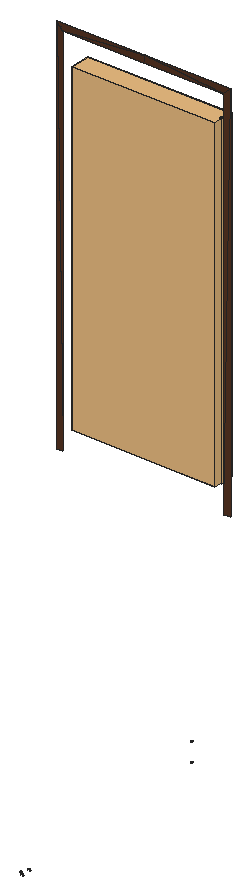
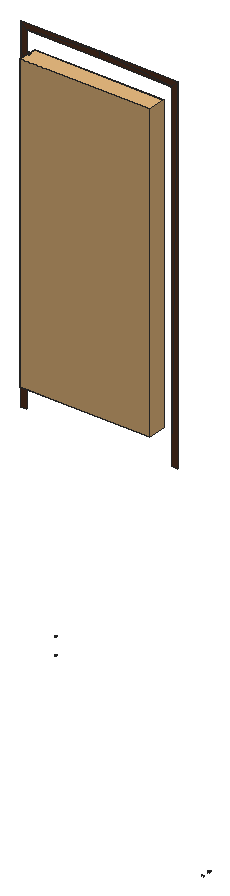
# SketchUp Ruby script. Lengths in inches.
U = 1.inch
M = Sketchup.active_model
def pt(a) = Geom::Point3d.new(a.map { |v| v * U })
def face(e, loops, mat)
  f = e.add_face(loops[0].map { |a| pt(a) })
  loops[1..].each { |l| e.add_face(l.map { |a| pt(a) }).erase! }
  f.material = f.back_material = mat if mat
  f
end
# faces: each face lists its corners as indices into pts; further lists are holes
def faces(e, pts, list, mat = nil) = list.each { |f| face(e, (f[0].is_a?(Array) ? f : [f]).map { |l| l.map { |i| pts[i] } }, mat) }
# xy, xz, yz: faces in a plane at the given z, y or x. An outline is a flat list of corners, or four numbers for a rectangle; further outlines are holes
def ring(l) = l.size == 4 ? [[l[0], l[1]], [l[2], l[1]], [l[2], l[3]], [l[0], l[3]]] : l.each_slice(2).to_a
def flat(e, list, mat, &to3) = list.each { |f| face(e, (f[0].is_a?(Array) ? f : [f]).map { |l| ring(l).map { |u, v| to3.(u, v) } }, mat) }
def xy(e, z, list, mat = nil) = flat(e, list, mat) { |x, y| [x, y, z] }
def xz(e, y, list, mat = nil) = flat(e, list, mat) { |x, z| [x, y, z] }
def yz(e, x, list, mat = nil) = flat(e, list, mat) { |y, z| [x, y, z] }
def lines(e, pts, list) = list.each { |a, b| e.add_line(pt(pts[a]), pt(pts[b])) }
# prism: a flat outline (further loops are holes) pulled along v
def prism(e, loops, v, mat = nil)
  f = face(e, loops, mat); d = Geom::Vector3d.new(v.map { |x| x * U })
  f.pushpull(f.normal.samedirection?(d) ? d.length : -d.length)
end
def box(e, o, s, mat = nil) = prism(e, [[o, [o[0] + s[0], o[1], o[2]], [o[0] + s[0], o[1] + s[1], o[2]], [o[0], o[1] + s[1], o[2]]]], [0, 0, s[2]], mat)
def at(x, y, z, deg = 0) = Geom::Transformation.translation(pt([x, y, z])) * Geom::Transformation.rotation(ORIGIN, Z_AXIS, deg.degrees)
def axes(o, x, y, z) = Geom::Transformation.new([*x, 0, *y, 0, *z, 0, *pt(o).to_a, 1])
def part(name) = M.definitions.add(name)
# library, detail: a bought-in or finely detailed component or shape, given as its bounding box
def library(name, o, s) = part(name).tap { |d| box(d.entities, o, s) }
def detail(e, o, s) = box(e.add_group.entities, o, s)
def put(e, d, t, mat = nil) = e.add_instance(d, t).tap { |i| i.material = mat if mat }
def group(e, t, mat = nil) = e.add_group.tap { |g| g.transformation = t; g.material = mat if mat }.entities
root = M.entities
M.materials.add("Material \#0").color = [86, 53, 35]
M.materials.add("Material \#1").color = [140, 140, 140]
c1 = library("3DGeom~9_Defintion",[456.52,-471.89,-18.89],[5.57,1000,5.49])
c2 = library("3DGeom~7_Defintion",[455.56,-471.94,-18.85],[5.55,1000,5.48])
c3 = part("3DGeom~8_Defintion")
xz(c3.entities,-471.94,[[458.125,-17.29,459.53,-16.11,457.73,-17.15],[458.125,-17.29,458.54,-17.29,459.53,-16.11],[458.54,-17.29,458.93,-17.15,459.53,-16.11],[457.73,-17.15,459.53,-16.11,457.42,-16.88],[458.93,-17.15,459.25,-16.88,459.53,-16.11],
  [457.42,-16.88,459.53,-16.11,457.21,-16.52],[459.25,-16.88,459.46,-16.52,459.53,-16.11],[457.21,-16.52,459.53,-16.11,457.14,-16.11],[457.14,-16.11,459.53,-16.11,457.21,-15.7],[459.53,-16.11,457.42,-15.34,457.21,-15.7],
  [459.53,-16.11,457.73,-15.07,457.42,-15.34],[459.53,-16.11,458.125,-14.93,457.73,-15.07],[459.53,-16.11,458.54,-14.93,458.125,-14.93],[459.53,-16.11,458.93,-15.07,458.54,-14.93],[459.53,-16.11,459.25,-15.34,458.93,-15.07],
  [459.53,-16.11,459.46,-15.7,459.25,-15.34]],"Material \#1")
xz(c3.entities,-416.39,[[458.125,-17.29,457.73,-17.15,459.53,-16.11],[458.125,-17.29,459.53,-16.11,458.54,-17.29],[458.54,-17.29,459.53,-16.11,458.93,-17.15],[457.73,-17.15,457.42,-16.88,459.53,-16.11],[458.93,-17.15,459.53,-16.11,459.25,-16.88],
  [457.42,-16.88,457.21,-16.52,459.53,-16.11],[459.25,-16.88,459.53,-16.11,459.46,-16.52],[457.21,-16.52,457.14,-16.11,459.53,-16.11],[457.14,-16.11,457.21,-15.7,459.53,-16.11],[459.53,-16.11,457.21,-15.7,457.42,-15.34],
  [459.53,-16.11,457.42,-15.34,457.73,-15.07],[459.53,-16.11,457.73,-15.07,458.125,-14.93],[459.53,-16.11,458.125,-14.93,458.54,-14.93],[459.53,-16.11,458.54,-14.93,458.93,-15.07],[459.53,-16.11,458.93,-15.07,459.25,-15.34],
  [459.53,-16.11,459.25,-15.34,459.46,-15.7]],"Material \#1")
xz(c3.entities,-27.5,[[458.125,-17.29,459.53,-16.11,457.73,-17.15],[458.125,-17.29,458.54,-17.29,459.53,-16.11],[458.54,-17.29,458.93,-17.15,459.53,-16.11],[457.73,-17.15,459.53,-16.11,457.42,-16.88],[458.93,-17.15,459.25,-16.88,459.53,-16.11],
  [457.42,-16.88,459.53,-16.11,457.21,-16.52],[459.25,-16.88,459.46,-16.52,459.53,-16.11],[457.21,-16.52,459.53,-16.11,457.14,-16.11],[457.14,-16.11,459.53,-16.11,457.21,-15.7],[459.53,-16.11,457.42,-15.34,457.21,-15.7],
  [459.53,-16.11,457.73,-15.07,457.42,-15.34],[459.53,-16.11,458.125,-14.93,457.73,-15.07],[459.53,-16.11,458.54,-14.93,458.125,-14.93],[459.53,-16.11,458.93,-15.07,458.54,-14.93],[459.53,-16.11,459.25,-15.34,458.93,-15.07],
  [459.53,-16.11,459.46,-15.7,459.25,-15.34]],"Material \#1")
xz(c3.entities,28.06,[[458.125,-17.29,457.73,-17.15,459.53,-16.11],[458.125,-17.29,459.53,-16.11,458.54,-17.29],[458.54,-17.29,459.53,-16.11,458.93,-17.15],[457.73,-17.15,457.42,-16.88,459.53,-16.11],[458.93,-17.15,459.53,-16.11,459.25,-16.88],
  [457.42,-16.88,457.21,-16.52,459.53,-16.11],[459.25,-16.88,459.53,-16.11,459.46,-16.52],[457.21,-16.52,457.14,-16.11,459.53,-16.11],[457.14,-16.11,457.21,-15.7,459.53,-16.11],[459.53,-16.11,457.21,-15.7,457.42,-15.34],
  [459.53,-16.11,457.42,-15.34,457.73,-15.07],[459.53,-16.11,457.73,-15.07,458.125,-14.93],[459.53,-16.11,458.125,-14.93,458.54,-14.93],[459.53,-16.11,458.54,-14.93,458.93,-15.07],[459.53,-16.11,458.93,-15.07,459.25,-15.34],
  [459.53,-16.11,459.25,-15.34,459.46,-15.7]],"Material \#1")
xz(c3.entities,472.5,[[458.125,-17.29,459.53,-16.11,457.73,-17.15],[458.125,-17.29,458.54,-17.29,459.53,-16.11],[458.54,-17.29,458.93,-17.15,459.53,-16.11],[457.73,-17.15,459.53,-16.11,457.42,-16.88],[458.93,-17.15,459.25,-16.88,459.53,-16.11],
  [457.42,-16.88,459.53,-16.11,457.21,-16.52],[459.25,-16.88,459.46,-16.52,459.53,-16.11],[457.21,-16.52,459.53,-16.11,457.14,-16.11],[457.14,-16.11,459.53,-16.11,457.21,-15.7],[459.53,-16.11,457.42,-15.34,457.21,-15.7],
  [459.53,-16.11,457.73,-15.07,457.42,-15.34],[459.53,-16.11,458.125,-14.93,457.73,-15.07],[459.53,-16.11,458.54,-14.93,458.125,-14.93],[459.53,-16.11,458.93,-15.07,458.54,-14.93],[459.53,-16.11,459.25,-15.34,458.93,-15.07],
  [459.53,-16.11,459.46,-15.7,459.25,-15.34]],"Material \#1")
xz(c3.entities,528.06,[[458.125,-17.29,457.73,-17.15,459.53,-16.11],[458.125,-17.29,459.53,-16.11,458.54,-17.29],[458.54,-17.29,459.53,-16.11,458.93,-17.15],[457.73,-17.15,457.42,-16.88,459.53,-16.11],[458.93,-17.15,459.53,-16.11,459.25,-16.88],
  [457.42,-16.88,457.21,-16.52,459.53,-16.11],[459.25,-16.88,459.53,-16.11,459.46,-16.52],[457.21,-16.52,457.14,-16.11,459.53,-16.11],[457.14,-16.11,457.21,-15.7,459.53,-16.11],[459.53,-16.11,457.21,-15.7,457.42,-15.34],
  [459.53,-16.11,457.42,-15.34,457.73,-15.07],[459.53,-16.11,457.73,-15.07,458.125,-14.93],[459.53,-16.11,458.125,-14.93,458.54,-14.93],[459.53,-16.11,458.54,-14.93,458.93,-15.07],[459.53,-16.11,458.93,-15.07,459.25,-15.34],
  [459.53,-16.11,459.25,-15.34,459.46,-15.7]],"Material \#1")
c4 = part("3DGeom~21_Defintion")
xy(c4.entities,73.08,[[-976.3,-241.71,23.7,-241.71,-976.3,-223.46],[23.7,-241.71,5.45,-223.46,-976.3,-223.46],[23.7,-241.71,23.7,0,5.45,-223.46],[5.45,-223.46,23.7,0,5.45,0],[23.7,0,23.7,241.71,5.45,223.46],
  [5.45,0,23.7,0,5.45,223.46],[-976.3,223.46,23.7,241.71,-976.3,241.71],[-976.3,223.46,5.45,223.46,23.7,241.71]],"Material \#0")
c5 = library("3DGeom~6_Defintion",[-5.59,-471.8,-48.03],[468.87,1000,73.72])
xy(root,78.84,[[381.98,199.78,381.91,199.8,381.92,199.81],[381.98,199.78,381.92,199.81,381.98,199.79],[381.98,199.78,381.98,199.79,382.05,199.78],[382.05,199.78,381.98,199.79,382.05,199.79],[382.05,199.78,382.05,199.79,382.12,199.8],
  [382.05,199.79,382.11,199.81,382.12,199.8],[381.91,199.8,381.86,199.83,381.87,199.84],[381.91,199.8,381.87,199.84,381.92,199.81],[382.12,199.8,382.11,199.81,382.17,199.83],[382.11,199.81,382.16,199.84,382.17,199.83],
  [381.86,199.83,381.82,199.88,381.84,199.88],[381.86,199.83,381.84,199.88,381.87,199.84],[382.17,199.83,382.16,199.84,382.21,199.88],[382.16,199.84,382.19,199.88,382.21,199.88],[381.82,199.88,381.81,199.93,381.83,199.93],
  [381.82,199.88,381.83,199.93,381.84,199.88],[382.19,199.88,382.2,199.93,382.22,199.93],[382.19,199.88,382.22,199.93,382.21,199.88],[381.81,199.93,381.82,199.98,381.84,199.98],[381.81,199.93,381.84,199.98,381.83,199.93],
  [382.2,199.93,382.19,199.98,382.21,199.98],[382.2,199.93,382.21,199.98,382.22,199.93],[381.82,199.98,381.86,200.03,381.87,200.02],[381.82,199.98,381.87,200.02,381.84,199.98],[382.19,199.98,382.16,200.02,382.17,200.03],
  [382.19,199.98,382.17,200.03,382.21,199.98],[381.87,200.02,381.86,200.03,381.92,200.05],[382.16,200.02,382.11,200.05,382.12,200.07],[382.16,200.02,382.12,200.07,382.17,200.03],[381.86,200.03,381.91,200.07,381.92,200.05],
  [381.92,200.05,381.91,200.07,381.98,200.07],[382.11,200.05,382.05,200.07,382.05,200.08],[382.11,200.05,382.05,200.08,382.12,200.07],[381.91,200.07,381.98,200.08,381.98,200.07],[381.98,200.07,381.98,200.08,382.05,200.07],
  [382.05,200.07,381.98,200.08,382.05,200.08]],"Material \#1")
xy(root,78.85,[[381.98,199.78,381.98,199.79,381.91,199.8],[381.98,199.78,382.05,199.78,382.05,199.79],[381.98,199.78,382.05,199.79,381.98,199.79],[382.05,199.78,382.11,199.81,382.05,199.79],[382.05,199.78,382.12,199.8,382.11,199.81],
  [381.98,199.79,381.92,199.81,381.91,199.8],[381.91,199.8,381.92,199.81,381.86,199.83],[382.12,199.8,382.16,199.84,382.11,199.81],[382.12,199.8,382.17,199.83,382.16,199.84],[381.92,199.81,381.87,199.84,381.86,199.83],
  [381.86,199.83,381.87,199.84,381.82,199.88],[382.17,199.83,382.19,199.88,382.16,199.84],[382.17,199.83,382.21,199.88,382.19,199.88],[381.87,199.84,381.84,199.88,381.82,199.88],[381.82,199.88,381.84,199.88,381.81,199.93],
  [381.84,199.88,381.83,199.93,381.81,199.93],[382.19,199.88,382.21,199.88,382.2,199.93],[382.21,199.88,382.22,199.93,382.2,199.93],[381.81,199.93,381.83,199.93,381.82,199.98],[381.83,199.93,381.84,199.98,381.82,199.98],
  [382.2,199.93,382.22,199.93,382.19,199.98],[382.22,199.93,382.21,199.98,382.19,199.98],[381.82,199.98,381.84,199.98,381.86,200.03],[381.84,199.98,381.87,200.02,381.86,200.03],[382.19,199.98,382.21,199.98,382.16,200.02],
  [382.21,199.98,382.17,200.03,382.16,200.02],[381.87,200.02,381.91,200.07,381.86,200.03],[381.87,200.02,381.92,200.05,381.91,200.07],[382.16,200.02,382.17,200.03,382.11,200.05],[382.17,200.03,382.12,200.07,382.11,200.05],
  [381.92,200.05,381.98,200.08,381.91,200.07],[381.92,200.05,381.98,200.07,381.98,200.08],[382.11,200.05,382.12,200.07,382.05,200.07],[381.98,200.07,382.05,200.07,382.05,200.08],[381.98,200.07,382.05,200.08,381.98,200.08],
  [382.05,200.07,382.12,200.07,382.05,200.08]],"Material \#1")
xy(root,82.67,[[381.98,199.78,381.91,199.8,381.98,199.79],[381.98,199.78,381.98,199.79,382.05,199.79],[381.98,199.78,382.05,199.79,382.05,199.78],[382.05,199.78,382.05,199.79,382.11,199.81],[382.05,199.78,382.11,199.81,382.12,199.8],
  [381.98,199.79,381.91,199.8,381.92,199.81],[381.91,199.8,381.86,199.83,381.92,199.81],[382.12,199.8,382.11,199.81,382.16,199.84],[382.12,199.8,382.16,199.84,382.17,199.83],[381.92,199.81,381.86,199.83,381.87,199.84],
  [381.86,199.83,381.82,199.88,381.87,199.84],[382.17,199.83,382.16,199.84,382.19,199.88],[382.17,199.83,382.19,199.88,382.21,199.88],[381.87,199.84,381.82,199.88,381.84,199.88],[381.82,199.88,381.81,199.93,381.84,199.88],
  [381.84,199.88,381.81,199.93,381.83,199.93],[382.19,199.88,382.2,199.93,382.21,199.88],[382.21,199.88,382.2,199.93,382.22,199.93],[381.81,199.93,381.82,199.98,381.83,199.93],[381.83,199.93,381.82,199.98,381.84,199.98],
  [382.2,199.93,382.19,199.98,382.22,199.93],[382.22,199.93,382.19,199.98,382.21,199.98],[381.82,199.98,381.86,200.03,381.84,199.98],[381.84,199.98,381.86,200.03,381.87,200.02],[382.19,199.98,382.16,200.02,382.21,199.98],
  [382.21,199.98,382.16,200.02,382.17,200.03],[381.87,200.02,381.86,200.03,381.91,200.07],[381.87,200.02,381.91,200.07,381.92,200.05],[382.16,200.02,382.11,200.05,382.17,200.03],[382.17,200.03,382.11,200.05,382.12,200.07],
  [381.92,200.05,381.91,200.07,381.98,200.08],[381.92,200.05,381.98,200.08,381.98,200.07],[382.11,200.05,382.05,200.07,382.12,200.07],[381.98,200.07,381.98,200.08,382.05,200.08],[381.98,200.07,382.05,200.08,382.05,200.07],
  [382.05,200.07,382.05,200.08,382.12,200.07]],"Material \#1")
xy(root,82.68,[[381.98,199.78,381.92,199.81,381.91,199.8],[381.98,199.78,381.98,199.79,381.92,199.81],[381.98,199.78,382.05,199.78,381.98,199.79],[382.05,199.78,382.05,199.79,381.98,199.79],[382.05,199.78,382.12,199.8,382.05,199.79],
  [382.05,199.79,382.12,199.8,382.11,199.81],[381.91,199.8,381.87,199.84,381.86,199.83],[381.91,199.8,381.92,199.81,381.87,199.84],[382.12,199.8,382.17,199.83,382.11,199.81],[382.11,199.81,382.17,199.83,382.16,199.84],
  [381.86,199.83,381.84,199.88,381.82,199.88],[381.86,199.83,381.87,199.84,381.84,199.88],[382.17,199.83,382.21,199.88,382.16,199.84],[382.16,199.84,382.21,199.88,382.19,199.88],[381.82,199.88,381.83,199.93,381.81,199.93],
  [381.82,199.88,381.84,199.88,381.83,199.93],[382.19,199.88,382.21,199.88,382.22,199.93],[382.19,199.88,382.22,199.93,382.2,199.93],[381.81,199.93,381.83,199.93,381.84,199.98],[381.81,199.93,381.84,199.98,381.82,199.98],
  [382.2,199.93,382.21,199.98,382.19,199.98],[382.2,199.93,382.22,199.93,382.21,199.98],[381.82,199.98,381.84,199.98,381.87,200.02],[381.82,199.98,381.87,200.02,381.86,200.03],[382.19,199.98,382.17,200.03,382.16,200.02],
  [382.19,199.98,382.21,199.98,382.17,200.03],[381.87,200.02,381.92,200.05,381.86,200.03],[382.16,200.02,382.12,200.07,382.11,200.05],[382.16,200.02,382.17,200.03,382.12,200.07],[381.86,200.03,381.92,200.05,381.91,200.07],
  [381.92,200.05,381.98,200.07,381.91,200.07],[382.11,200.05,382.05,200.08,382.05,200.07],[382.11,200.05,382.12,200.07,382.05,200.08],[381.91,200.07,381.98,200.07,381.98,200.08],[381.98,200.07,382.05,200.07,381.98,200.08],
  [382.05,200.07,382.05,200.08,381.98,200.08]],"Material \#1")
xy(root,131.7,[[388.01,199.78,387.96,199.8,387.97,199.81],[388.01,199.78,387.97,199.81,388.02,199.79],[388.01,199.78,388.02,199.79,388.07,199.78],[388.07,199.78,388.02,199.79,388.07,199.79],[388.07,199.78,388.07,199.79,388.13,199.8],
  [388.07,199.79,388.12,199.81,388.13,199.8],[387.96,199.8,387.91,199.83,387.92,199.84],[387.96,199.8,387.92,199.84,387.97,199.81],[388.13,199.8,388.12,199.81,388.18,199.83],[388.12,199.81,388.16,199.84,388.18,199.83],
  [387.91,199.83,387.88,199.88,387.9,199.88],[387.91,199.83,387.9,199.88,387.92,199.84],[388.18,199.83,388.16,199.84,388.21,199.88],[388.16,199.84,388.19,199.88,388.21,199.88],[387.88,199.88,387.87,199.93,387.89,199.93],
  [387.88,199.88,387.89,199.93,387.9,199.88],[388.19,199.88,388.2,199.93,388.22,199.93],[388.19,199.88,388.22,199.93,388.21,199.88],[387.87,199.93,387.88,199.98,387.9,199.98],[387.87,199.93,387.9,199.98,387.89,199.93],
  [388.2,199.93,388.19,199.98,388.21,199.98],[388.2,199.93,388.21,199.98,388.22,199.93],[387.88,199.98,387.91,200.03,387.92,200.02],[387.88,199.98,387.92,200.02,387.9,199.98],[388.19,199.98,388.16,200.02,388.18,200.03],
  [388.19,199.98,388.18,200.03,388.21,199.98],[387.92,200.02,387.91,200.03,387.97,200.05],[388.16,200.02,388.12,200.05,388.13,200.07],[388.16,200.02,388.13,200.07,388.18,200.03],[387.91,200.03,387.96,200.07,387.97,200.05],
  [387.97,200.05,387.96,200.07,388.02,200.07],[388.12,200.05,388.07,200.07,388.07,200.08],[388.12,200.05,388.07,200.08,388.13,200.07],[387.96,200.07,388.01,200.08,388.02,200.07],[388.02,200.07,388.01,200.08,388.07,200.07],
  [388.07,200.07,388.01,200.08,388.07,200.08]],"Material \#1")
xy(root,131.72,[[388.01,199.78,388.02,199.79,387.96,199.8],[388.01,199.78,388.07,199.78,388.07,199.79],[388.01,199.78,388.07,199.79,388.02,199.79],[388.07,199.78,388.12,199.81,388.07,199.79],[388.07,199.78,388.13,199.8,388.12,199.81],
  [388.02,199.79,387.97,199.81,387.96,199.8],[387.96,199.8,387.97,199.81,387.91,199.83],[388.13,199.8,388.16,199.84,388.12,199.81],[388.13,199.8,388.18,199.83,388.16,199.84],[387.97,199.81,387.92,199.84,387.91,199.83],
  [387.91,199.83,387.92,199.84,387.88,199.88],[388.18,199.83,388.19,199.88,388.16,199.84],[388.18,199.83,388.21,199.88,388.19,199.88],[387.92,199.84,387.9,199.88,387.88,199.88],[387.88,199.88,387.9,199.88,387.87,199.93],
  [387.9,199.88,387.89,199.93,387.87,199.93],[388.19,199.88,388.21,199.88,388.2,199.93],[388.21,199.88,388.22,199.93,388.2,199.93],[387.87,199.93,387.89,199.93,387.88,199.98],[387.89,199.93,387.9,199.98,387.88,199.98],
  [388.2,199.93,388.22,199.93,388.19,199.98],[388.22,199.93,388.21,199.98,388.19,199.98],[387.88,199.98,387.9,199.98,387.91,200.03],[387.9,199.98,387.92,200.02,387.91,200.03],[388.19,199.98,388.21,199.98,388.16,200.02],
  [388.21,199.98,388.18,200.03,388.16,200.02],[387.92,200.02,387.96,200.07,387.91,200.03],[387.92,200.02,387.97,200.05,387.96,200.07],[388.16,200.02,388.18,200.03,388.12,200.05],[388.18,200.03,388.13,200.07,388.12,200.05],
  [387.97,200.05,388.01,200.08,387.96,200.07],[387.97,200.05,388.02,200.07,388.01,200.08],[388.12,200.05,388.13,200.07,388.07,200.07],[388.02,200.07,388.07,200.08,388.01,200.08],[388.02,200.07,388.07,200.07,388.07,200.08],
  [388.07,200.07,388.13,200.07,388.07,200.08]],"Material \#1")
xy(root,135.01,[[388.01,199.78,387.96,199.8,388.02,199.79],[388.01,199.78,388.02,199.79,388.07,199.79],[388.01,199.78,388.07,199.79,388.07,199.78],[388.07,199.78,388.07,199.79,388.12,199.81],[388.07,199.78,388.12,199.81,388.13,199.8],
  [388.02,199.79,387.96,199.8,387.97,199.81],[387.96,199.8,387.91,199.83,387.97,199.81],[388.13,199.8,388.12,199.81,388.16,199.84],[388.13,199.8,388.16,199.84,388.18,199.83],[387.97,199.81,387.91,199.83,387.92,199.84],
  [387.91,199.83,387.88,199.88,387.92,199.84],[388.18,199.83,388.16,199.84,388.19,199.88],[388.18,199.83,388.19,199.88,388.21,199.88],[387.92,199.84,387.88,199.88,387.9,199.88],[387.88,199.88,387.87,199.93,387.9,199.88],
  [387.9,199.88,387.87,199.93,387.89,199.93],[388.19,199.88,388.2,199.93,388.21,199.88],[388.21,199.88,388.2,199.93,388.22,199.93],[387.87,199.93,387.88,199.98,387.89,199.93],[387.89,199.93,387.88,199.98,387.9,199.98],
  [388.2,199.93,388.19,199.98,388.22,199.93],[388.22,199.93,388.19,199.98,388.21,199.98],[387.88,199.98,387.91,200.03,387.9,199.98],[387.9,199.98,387.91,200.03,387.92,200.02],[388.19,199.98,388.16,200.02,388.21,199.98],
  [388.21,199.98,388.16,200.02,388.18,200.03],[387.92,200.02,387.91,200.03,387.96,200.07],[387.92,200.02,387.96,200.07,387.97,200.05],[388.16,200.02,388.12,200.05,388.18,200.03],[388.18,200.03,388.12,200.05,388.13,200.07],
  [387.97,200.05,387.96,200.07,388.01,200.08],[387.97,200.05,388.01,200.08,388.02,200.07],[388.12,200.05,388.07,200.07,388.13,200.07],[388.02,200.07,388.01,200.08,388.07,200.08],[388.02,200.07,388.07,200.08,388.07,200.07],
  [388.07,200.07,388.07,200.08,388.13,200.07]],"Material \#1")
xy(root,135.03,[[388.01,199.78,387.97,199.81,387.96,199.8],[388.01,199.78,388.02,199.79,387.97,199.81],[388.01,199.78,388.07,199.78,388.02,199.79],[388.07,199.78,388.07,199.79,388.02,199.79],[388.07,199.78,388.13,199.8,388.07,199.79],
  [388.07,199.79,388.13,199.8,388.12,199.81],[387.96,199.8,387.92,199.84,387.91,199.83],[387.96,199.8,387.97,199.81,387.92,199.84],[388.13,199.8,388.18,199.83,388.12,199.81],[388.12,199.81,388.18,199.83,388.16,199.84],
  [387.91,199.83,387.9,199.88,387.88,199.88],[387.91,199.83,387.92,199.84,387.9,199.88],[388.18,199.83,388.21,199.88,388.16,199.84],[388.16,199.84,388.21,199.88,388.19,199.88],[387.88,199.88,387.89,199.93,387.87,199.93],
  [387.88,199.88,387.9,199.88,387.89,199.93],[388.19,199.88,388.21,199.88,388.22,199.93],[388.19,199.88,388.22,199.93,388.2,199.93],[387.87,199.93,387.89,199.93,387.9,199.98],[387.87,199.93,387.9,199.98,387.88,199.98],
  [388.2,199.93,388.21,199.98,388.19,199.98],[388.2,199.93,388.22,199.93,388.21,199.98],[387.88,199.98,387.9,199.98,387.92,200.02],[387.88,199.98,387.92,200.02,387.91,200.03],[388.19,199.98,388.18,200.03,388.16,200.02],
  [388.19,199.98,388.21,199.98,388.18,200.03],[387.92,200.02,387.97,200.05,387.91,200.03],[388.16,200.02,388.13,200.07,388.12,200.05],[388.16,200.02,388.18,200.03,388.13,200.07],[387.91,200.03,387.97,200.05,387.96,200.07],
  [387.97,200.05,388.02,200.07,387.96,200.07],[388.12,200.05,388.07,200.08,388.07,200.07],[388.12,200.05,388.13,200.07,388.07,200.08],[387.96,200.07,388.02,200.07,388.01,200.08],[388.02,200.07,388.07,200.07,388.01,200.08],
  [388.07,200.07,388.07,200.08,388.01,200.08]],"Material \#1")
xz(root,199.31,[[348.54,46.74,348.52,46.875,348.55,46.74],[348.55,46.74,348.52,46.875,348.54,46.88],[348.52,46.875,348.49,47,348.54,46.88],[348.01,46.88,348.02,46.92,348.03,46.92],[348.54,46.88,348.49,47,348.5,47],
  [348.02,46.92,348.04,46.96,348.03,46.92],[348.03,46.92,348.04,46.96,348.05,46.95],[348.05,46.95,348.04,46.96,348.05,47],[348.05,46.95,348.05,47,348.0625,47],[348.05,47,348.05,47.04,348.0625,47],
  [348.0625,47,348.05,47.04,348.06,47.04],[348.49,47,348.4375,47.11,348.5,47],[348.5,47,348.4375,47.11,348.45,47.12],[348.05,47.04,348.05,47.08,348.06,47.04],[348.06,47.04,348.05,47.08,348.0625,47.09],
  [348.05,47.08,348.04,47.12,348.0625,47.09],[348.0625,47.09,348.04,47.12,348.05,47.13],[348.4375,47.11,348.37,47.21,348.45,47.12],[348.04,47.12,348.02,47.16,348.05,47.13],[348.45,47.12,348.37,47.21,348.38,47.22],
  [348.05,47.13,348.02,47.16,348.03,47.17],[348.02,47.16,348,47.19,348.03,47.17],[348.03,47.17,348,47.19,348.01,47.2],[348,47.19,347.97,47.22,348.01,47.2],[348.01,47.2,347.97,47.22,347.98,47.23],
  [348.37,47.21,348.28,47.3,348.38,47.22],[347.97,47.22,347.9375,47.24,347.98,47.23],[348.38,47.22,348.28,47.3,348.29,47.3125],[347.98,47.23,347.9375,47.24,347.95,47.25],[347.9375,47.24,347.9,47.26,347.95,47.25],
  [348.28,47.3,348.18,47.375,348.29,47.3125],[348.07,47.43,347.95,47.46,348.08,47.44],[348.08,47.44,347.95,47.46,347.95,47.47]],"Material \#1")
xz(root,201.11,[[348.49,47,348.5,47,348.4375,47.11],[348.5,47,348.45,47.12,348.4375,47.11],[348.05,47.04,348.06,47.04,348.05,47.08],[348.4375,47.11,348.45,47.12,348.37,47.21],[348.45,47.12,348.38,47.22,348.37,47.21]],"Material \#1")
put(root,c1,axes([359.55,200.83,162.74],[0.06203,0,0],[0,0,0.06599],[0,0.05589,0]),"Material \#1")
put(root,c2,axes([359.55,200.83,162.74],[0.06217,0,0],[0,0,0.06613],[0,0.05601,0]),"Material \#1")
put(root,c3,axes([359.55,200.83,162.74],[0.06217,0,0],[0,0,0.06613],[0,0.05601,0]),"Material \#1")
put(root,c4,axes([372.33,204.75,201.6875],[0,0,0.07752],[0.07287,0,0],[0,-0.06565,0]),"Material \#0")
put(root,c5,axes([359.55,200.83,162.74],[0.06184,0,0],[0,0,0.06578],[0,0.05571,0]),"Material \#1")
